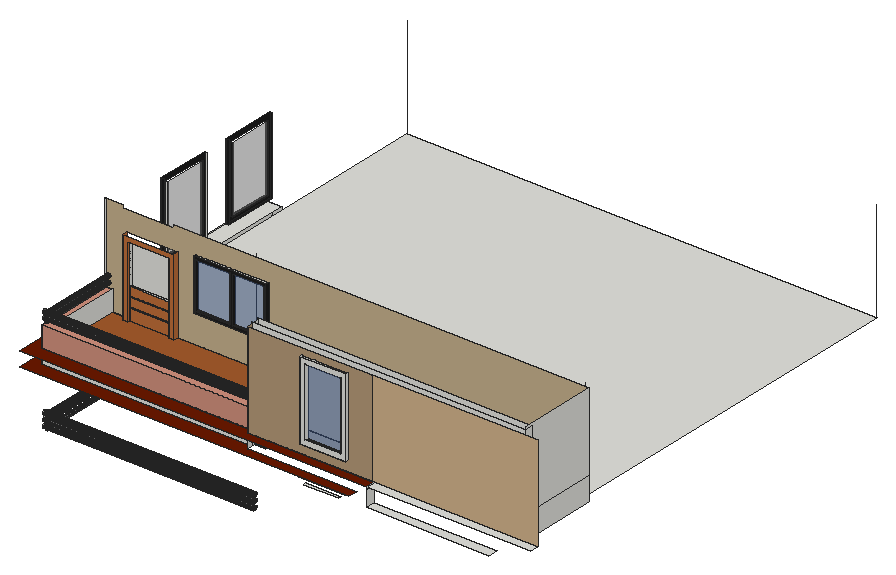
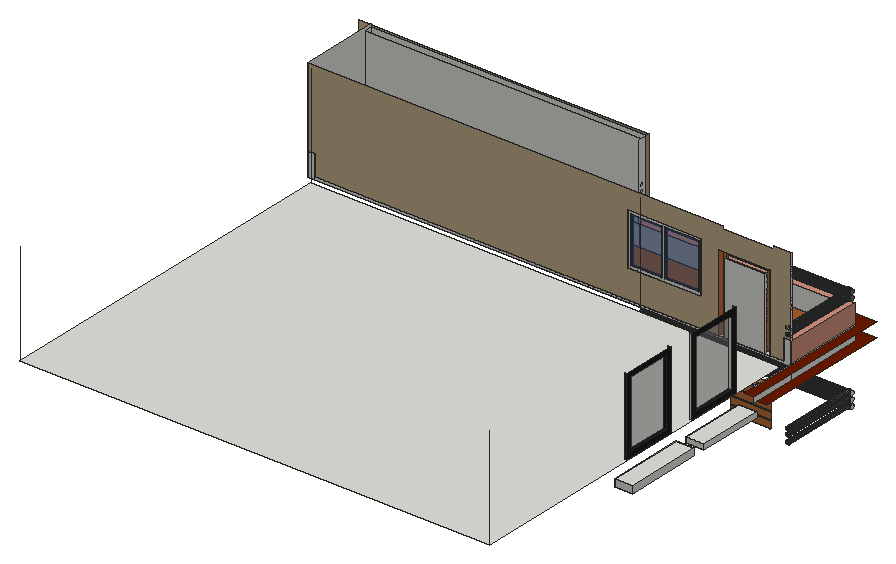
# SketchUp Ruby script. Lengths in inches.
U = 1.inch
M = Sketchup.active_model
def pt(a) = Geom::Point3d.new(a.map { |v| v * U })
def face(e, loops, mat)
  f = e.add_face(loops[0].map { |a| pt(a) })
  loops[1..].each { |l| e.add_face(l.map { |a| pt(a) }).erase! }
  f.material = f.back_material = mat if mat
  f
end
# faces: each face lists its corners as indices into pts; further lists are holes
def faces(e, pts, list, mat = nil) = list.each { |f| face(e, (f[0].is_a?(Array) ? f : [f]).map { |l| l.map { |i| pts[i] } }, mat) }
# xy, xz, yz: faces in a plane at the given z, y or x. An outline is a flat list of corners, or four numbers for a rectangle; further outlines are holes
def ring(l) = l.size == 4 ? [[l[0], l[1]], [l[2], l[1]], [l[2], l[3]], [l[0], l[3]]] : l.each_slice(2).to_a
def flat(e, list, mat, &to3) = list.each { |f| face(e, (f[0].is_a?(Array) ? f : [f]).map { |l| ring(l).map { |u, v| to3.(u, v) } }, mat) }
def xy(e, z, list, mat = nil) = flat(e, list, mat) { |x, y| [x, y, z] }
def xz(e, y, list, mat = nil) = flat(e, list, mat) { |x, z| [x, y, z] }
def yz(e, x, list, mat = nil) = flat(e, list, mat) { |y, z| [x, y, z] }
def lines(e, pts, list) = list.each { |a, b| e.add_line(pt(pts[a]), pt(pts[b])) }
# prism: a flat outline (further loops are holes) pulled along v
def prism(e, loops, v, mat = nil)
  f = face(e, loops, mat); d = Geom::Vector3d.new(v.map { |x| x * U })
  f.pushpull(f.normal.samedirection?(d) ? d.length : -d.length)
end
def box(e, o, s, mat = nil) = prism(e, [[o, [o[0] + s[0], o[1], o[2]], [o[0] + s[0], o[1] + s[1], o[2]], [o[0], o[1] + s[1], o[2]]]], [0, 0, s[2]], mat)
def at(x, y, z, deg = 0) = Geom::Transformation.translation(pt([x, y, z])) * Geom::Transformation.rotation(ORIGIN, Z_AXIS, deg.degrees)
def axes(o, x, y, z) = Geom::Transformation.new([*x, 0, *y, 0, *z, 0, *pt(o).to_a, 1])
def part(name) = M.definitions.add(name)
# library, detail: a bought-in or finely detailed component or shape, given as its bounding box
def library(name, o, s) = part(name).tap { |d| box(d.entities, o, s) }
def detail(e, o, s) = box(e.add_group.entities, o, s)
def put(e, d, t, mat = nil) = e.add_instance(d, t).tap { |i| i.material = mat if mat }
def group(e, t, mat = nil) = e.add_group.tap { |g| g.transformation = t; g.material = mat if mat }.entities
root = M.entities
M.materials.add("[0032_Moccasin]").color = [198, 177, 141]
M.materials.add("[0035_Tan]").color = [181, 154, 120]
M.materials.add("[0035_Tan]1").color = [210, 180, 140]
M.materials.add("[0134_DimGray]").color = [105, 105, 105]
M.materials.add("[Color B02]").color = [209, 145, 125]
M.materials.add("[Color B07]").color = [107, 26, 0]
M.materials.add("[Color M08]").color = [30, 30, 30]
M.materials.add("[Translucent Glass Blue]").color = [61, 91, 145]
M.materials["[Translucent Glass Blue]"].alpha = 0.5
M.materials.add("[Translucent Glass Gray]").color = [128, 128, 128]
M.materials["[Translucent Glass Gray]"].alpha = 0.5
M.materials.add("[Wood Square Tile 01]").color = [164, 91, 44]
M.materials.add("[Wood Veneer 01]").color = [191, 111, 58]
xy(root,293.5,[[141.33,116.9375,227.02,119.9375]],"[Color M08]")
xy(root,296.5,[[144.33,116.9375,184.18,119.9375],[187.18,116.9375,224.02,119.9375]],"[Color M08]")
xy(root,333,[[61.4,116.9375,109.4,119.9375]])
xy(root,333,[[61.4,113.9375,109.4,116.9375]],"[Wood Veneer 01]")
xy(root,339,[[55.4,113.9375,115.4,119.9375]],"[Wood Veneer 01]")
xy(root,342.9,[[350.26,17.9375,391.95,20.9375]])
xy(root,348.9,[[344.26,17.9375,397.95,20.9375]])
xy(root,350.47,[[430.625,9.86,574.78,20.9375]])
xy(root,351.1875,[[144.33,116.9375,184.18,119.9375],[187.18,116.9375,224.02,119.9375]],"[Color M08]")
xy(root,351.43,[[31.875,209.04,34.875,261.16],[31.875,307.48,34.875,359.6]],"[Color M08]")
xy(root,354.1875,[[141.33,116.9375,227.02,119.9375]],"[Color M08]")
xy(root,355.125,[[23.625,9.86,23.625,170.67,34.875,170.67,34.875,26.9375,282.125,26.9375,282.125,20.9375,410.07,20.9375,410.07,9.86]],"[Color B07]")
xy(root,357.43,[[13.875,198.04,13.875,275.26,34.875,275.26,34.875,267.16,31.875,267.16,31.875,203.04,34.875,203.04,34.875,198.04],[31.875,203.04,34.875,203.1],[31.875,203.1,34.875,267.16],[13.875,289.98,13.875,380.29,34.875,380.29,34.875,365.6,31.875,365.6,31.875,301.48,34.875,301.48,34.875,289.98],[31.875,301.48,34.875,365.6]])
xy(root,363.74,[[13.875,198.04,34.875,275.26]])
xy(root,365.49,[[13.875,289.98,34.875,380.29]])
xy(root,369,[[34.875,26.9375,34.875,119.9375,604.125,119.9375,604.125,35.9375,282.125,35.9375,282.125,26.9375],[282.125,26.9375,604.125,35.9375],[43.875,125.9375,595.125,552.98]])
xy(root,372,[[430.625,9.86,623,20.9375],[60.43,113.9375,66.43,119.9375],[114.43,113.9375,120.43,119.9375],[66.43,116.9375,114.43,119.9375]])
xy(root,372,[[23.625,9.86,430.625,9.86,430.625,20.9375,282.125,20.9375,282.125,26.9375,34.875,26.9375,34.875,189.6875,23.625,189.6875]],"[Color B07]")
xy(root,372,[[43.875,35.9375,595.125,35.9375,595.125,119.9375,120.43,119.9375,120.43,113.9375,114.43,113.9375,114.43,116.9375,66.43,116.9375,66.43,113.9375,60.43,113.9375,60.43,119.9375,43.875,119.9375]],"[Wood Square Tile 01]")
xy(root,380.37,[[31.875,206.29,34.875,270.41]])
xy(root,380.37,[[31.875,301.48,34.875,365.6]],"[Color M08]")
xy(root,384.33,[[346.1,17.9375,399.78,20.9375]])
xy(root,386.37,[[31.875,212.29,34.875,264.41],[31.875,307.48,34.875,359.6]],"[Color M08]")
xy(root,390.33,[[352.1,17.9375,393.78,20.9375]])
xy(root,396,[[282.125,26.9375,604.125,35.9375],[595.125,35.9375,604.125,119.9375]])
xy(root,396,[[34.875,26.9375,282.125,26.9375,282.125,35.9375,43.875,35.9375,43.875,119.9375,34.875,119.9375]],"[Color B02]")
xy(root,406.125,[[141.33,116.9375,227.02,119.9375]])
xy(root,409.125,[[144.33,116.9375,184.18,119.9375],[187.18,116.9375,224.02,119.9375]],"[Color M08]")
xz(root,17.9375,[[[346.1,384.33,399.78,476.15],[352.1,390.33,393.78,470.15]]])
xz(root,20.9375,[[282.125,369,430.625,372],[[346.1,384.33,399.78,476.15],[352.1,390.33,393.78,470.15]]])
xz(root,20.9375,[[[282.125,372,427.625,483.875],[346.1,384.33,399.78,476.15]]],"[0035_Tan]")
xz(root,20.9375,[[427.625,372,623,483.875]],"[0035_Tan]1")
xz(root,20.9375,[[352.1,390.33,393.78,470.15]],"[Translucent Glass Blue]")
xz(root,26.9375,[[34.875,355.125,282.125,369],[34.875,369,282.125,372],[282.125,369,604.125,396],[282.125,396,604.125,485.875]])
xz(root,26.9375,[[34.875,372,282.125,396]],"[Color B02]")
xz(root,29.25,[[39.51,399.11,40.12,399.19,40.69,399.43,41.1875,399.81,41.5625,400.3,41.8,400.87,41.88,401.49,41.8,402.1,41.5625,402.67,41.1875,403.17,40.69,403.54,40.12,403.78,39.51,403.86,38.89,403.78,38.32,403.54,37.83,403.17,37.45,402.67,37.21,402.1,37.13,401.49,37.21,400.87,37.45,400.3,37.83,399.81,38.32,399.43,38.89,399.19]])
xz(root,35.9375,[[43.875,372,282.125,396],[282.125,372,595.125,396],[282.125,396,604.125,485.875]])
xz(root,113.9375,[[60.43,372,66.43,372,66.43,456,114.43,456,114.43,372,120.43,372,120.43,462,60.43,462]],"[Wood Veneer 01]")
xz(root,116.9375,[[61.4,292.58,109.4,293.56],[61.4,301.83,109.4,302.81],[61.4,311.08,109.4,312.06],[61.4,320.33,109.4,321.31],[66.43,385.34,114.43,387.06],
  [66.43,396.78,114.43,398.5],[66.43,408.22,114.43,409.93]])
xz(root,116.9375,[[[141.33,293.5,227.02,354.1875],[144.33,296.5,184.18,351.1875],[187.18,296.5,224.02,351.1875]],[[141.33,406.125,227.02,466.8125],[144.33,409.125,184.18,463.8125],[187.18,409.125,224.02,463.8125]]],"[Color M08]")
xz(root,116.9375,[[61.4,293.56,109.4,301.83],[61.4,302.81,109.4,311.08],[61.4,312.06,109.4,320.33],[61.4,321.31,109.4,333],[66.43,372,114.43,385.34],
  [66.43,387.06,114.43,396.78],[66.43,398.5,114.43,408.22]],"[Wood Veneer 01]")
xz(root,119.9375,[[[141.33,293.5,227.02,354.1875],[144.33,296.5,184.18,351.1875],[187.18,296.5,224.02,351.1875]],[34.875,369,35.6,396],[35.6,369,60.43,369,60.43,372,43.875,372,43.875,396,35.6,396],[60.43,369,120.43,372],[120.43,369,595.125,372],
  [595.125,369,604.125,396],[66.43,372,114.43,456],[34.875,396,35.6,489],[[141.33,406.125,227.02,466.8125],[144.33,409.125,184.18,463.8125],[187.18,409.125,224.02,463.8125]]])
xz(root,119.9375,[[[43.875,372,60.43,372,60.43,462,120.43,462,120.43,372,595.125,372,595.125,396,604.125,396,604.125,489,116.21,489,116.21,486,56.21,486,56.21,489,35.6,489,35.6,396,43.875,396],[141.33,406.125,227.02,466.8125],[39.51,399.11,38.89,399.19,38.32,399.43,37.83,399.81,37.45,400.3,37.21,400.87,37.13,401.49,37.21,402.1,37.45,402.67,37.83,403.17,38.32,403.54,38.89,403.78,39.51,403.86,40.12,403.78,40.69,403.54,41.1875,403.17,41.5625,402.67,41.8,402.1,41.88,401.49,41.8,400.87,41.5625,400.3,41.1875,399.81,40.69,399.43,40.12,399.19]]],"[0032_Moccasin]")
xz(root,119.9375,[[144.33,296.5,184.18,351.1875],[187.18,296.5,224.02,351.1875],[144.33,409.125,184.18,463.8125],[187.18,409.125,224.02,463.8125]],"[Translucent Glass Blue]")
xz(root,198.04,[[13.875,357.43,34.875,363.74]])
xz(root,206.29,[[31.875,380.37,34.875,470.8]],"[Color M08]")
xz(root,212.29,[[31.875,386.37,34.875,464.8]])
xz(root,264.41,[[31.875,386.37,34.875,464.8]],"[Color M08]")
xz(root,270.41,[[31.875,380.37,34.875,470.8]])
xz(root,275.26,[[13.875,357.43,34.875,363.74]])
xz(root,289.98,[[13.875,357.43,34.875,365.49]])
xz(root,301.48,[[31.875,380.37,34.875,470.8]],"[Color M08]")
xz(root,307.48,[[31.875,386.37,34.875,464.8]],"[Color M08]")
xz(root,359.6,[[31.875,386.37,34.875,464.8]],"[Color M08]")
xz(root,365.6,[[31.875,380.37,34.875,470.8]],"[Color M08]")
xz(root,380.29,[[13.875,357.43,34.875,365.49]])
yz(root,13.875,[[198.04,357.43,275.26,363.74],[289.98,357.43,380.29,365.49]])
yz(root,31.875,[[[206.29,380.37,270.41,470.8],[212.29,386.37,264.41,464.8]],[[301.48,380.37,365.6,470.8],[307.48,386.37,359.6,464.8]]],"[Color M08]")
yz(root,34.875,[[31.46,285.87,30.85,285.95,30.27,286.1875,29.78,286.5625,29.4,287.06,29.17,287.63,29.09,288.24,29.17,288.86,29.4,289.43,29.78,289.92,30.27,290.3,30.85,290.54,31.46,290.62,32.08,290.54,32.65,290.3,33.14,289.92,33.52,289.43,33.76,288.86,33.84,288.24,33.76,287.63,33.52,287.06,33.14,286.5625,32.65,286.1875,32.08,285.95],[31.46,292.87,30.85,292.95,30.27,293.1875,29.78,293.5625,29.4,294.06,29.17,294.63,29.09,295.24,29.17,295.86,29.4,296.43,29.78,296.92,30.27,297.3,30.85,297.54,31.46,297.62,32.08,297.54,32.65,297.3,33.14,296.92,33.52,296.43,33.76,295.86,33.84,295.24,33.76,294.63,33.52,294.06,33.14,293.5625,32.65,293.1875,32.08,292.95],[31.46,299.87,30.85,299.95,30.27,300.1875,29.78,300.5625,29.4,301.06,29.17,301.63,29.09,302.24,29.17,302.86,29.4,303.43,29.78,303.92,30.27,304.3,30.85,304.54,31.46,304.62,32.08,304.54,32.65,304.3,33.14,303.92,33.52,303.43,33.76,302.86,33.84,302.24,33.76,301.63,33.52,301.06,33.14,300.5625,32.65,300.1875,32.08,299.95],[26.9375,355.125,119.9375,369],[119.9375,355.125,175.54,369],
  [198.04,357.43,203.1,363.74],[203.1,357.43,275.26,363.74],[289.98,357.43,365.6,365.49],[365.6,357.43,380.29,365.49],[26.9375,369,119.9375,372],
  [119.9375,369,175.54,372]])
yz(root,34.875,[[31.46,399.68,30.85,399.76,30.27,400,29.78,400.375,29.4,400.87,29.17,401.44,29.09,402.06,29.17,402.67,29.4,403.24,29.78,403.73,30.27,404.11,30.85,404.35,31.46,404.43,32.08,404.35,32.65,404.11,33.14,403.73,33.52,403.24,33.76,402.67,33.84,402.06,33.76,401.44,33.52,400.87,33.14,400.375,32.65,400,32.08,399.76],[31.46,406.37,30.85,406.45,30.27,406.6875,29.78,407.0625,29.4,407.56,29.17,408.13,29.09,408.74,29.17,409.36,29.4,409.93,29.78,410.42,30.27,410.8,30.85,411.04,31.46,411.12,32.08,411.04,32.65,410.8,33.14,410.42,33.52,409.93,33.76,409.36,33.84,408.74,33.76,408.13,33.52,407.56,33.14,407.0625,32.65,406.6875,32.08,406.45]],"[0134_DimGray]")
yz(root,34.875,[[26.9375,372,119.9375,396]],"[Color B02]")
yz(root,34.875,[[212.29,386.37,264.41,464.8],[307.48,386.37,359.6,464.8]],"[Translucent Glass Gray]")
yz(root,43.875,[[35.9375,372,119.9375,396]])
yz(root,60.43,[[113.9375,372,119.9375,462]],"[Wood Veneer 01]")
yz(root,66.43,[[116.9375,372,119.9375,456]])
yz(root,66.43,[[113.9375,372,116.9375,456]],"[Wood Veneer 01]")
yz(root,114.43,[[116.9375,372,119.9375,456]])
yz(root,114.43,[[113.9375,372,116.9375,456]],"[Wood Veneer 01]")
yz(root,120.43,[[113.9375,372,119.9375,462]],"[Wood Veneer 01]")
yz(root,141.33,[[116.9375,293.5,119.9375,354.1875]])
yz(root,141.33,[[116.9375,406.125,119.9375,466.8125]],"[Color M08]")
yz(root,144.33,[[116.9375,296.5,119.9375,351.1875],[116.9375,409.125,119.9375,463.8125]],"[Color M08]")
yz(root,184.18,[[116.9375,296.5,119.9375,351.1875],[116.9375,409.125,119.9375,463.8125]],"[Color M08]")
yz(root,187.18,[[116.9375,296.5,119.9375,351.1875],[116.9375,409.125,119.9375,463.8125]],"[Color M08]")
yz(root,224.02,[[116.9375,296.5,119.9375,351.1875],[116.9375,409.125,119.9375,463.8125]],"[Color M08]")
yz(root,227.02,[[116.9375,293.5,119.9375,354.1875],[116.9375,406.125,119.9375,466.8125]],"[Color M08]")
yz(root,282.125,[[20.9375,355.125,26.9375,369],[26.9375,355.125,35.9375,369],[20.9375,369,26.9375,372],[[26.9375,396,35.9375,483.875],[31.46,399.68,32.08,399.76,32.65,400,33.14,400.375,33.52,400.87,33.76,401.44,33.84,402.06,33.76,402.67,33.52,403.24,33.14,403.73,32.65,404.11,32.08,404.35,31.46,404.43,30.85,404.35,30.27,404.11,29.78,403.73,29.4,403.24,29.17,402.67,29.09,402.06,29.17,401.44,29.4,400.87,29.78,400.375,30.27,400,30.85,399.76],[31.46,406.37,32.08,406.45,32.65,406.6875,33.14,407.0625,33.52,407.56,33.76,408.13,33.84,408.74,33.76,409.36,33.52,409.93,33.14,410.42,32.65,410.8,32.08,411.04,31.46,411.12,30.85,411.04,30.27,410.8,29.78,410.42,29.4,409.93,29.17,409.36,29.09,408.74,29.17,408.13,29.4,407.56,29.78,407.0625,30.27,406.6875,30.85,406.45],[31.46,413.06,32.08,413.14,32.65,413.375,33.14,413.75,33.52,414.24,33.76,414.82,33.84,415.43,33.76,416.04,33.52,416.62,33.14,417.11,32.65,417.49,32.08,417.72,31.46,417.81,30.85,417.72,30.27,417.49,29.78,417.11,29.4,416.62,29.17,416.04,29.09,415.43,29.17,414.82,29.4,414.24,29.78,413.75,30.27,413.375,30.85,413.14],[31.46,419.74,32.08,419.82,32.65,420.0625,33.14,420.4375,33.52,420.93,33.76,421.5,33.84,422.12,33.76,422.73,33.52,423.31,33.14,423.8,32.65,424.17,32.08,424.41,31.46,424.49,30.85,424.41,30.27,424.17,29.78,423.8,29.4,423.31,29.17,422.73,29.09,422.12,29.17,421.5,29.4,420.93,29.78,420.4375,30.27,420.0625,30.85,419.82],[31.46,426.43,32.08,426.51,32.65,426.75,33.14,427.125,33.52,427.62,33.76,428.19,33.84,428.81,33.76,429.42,33.52,429.99,33.14,430.48,32.65,430.86,32.08,431.1,31.46,431.18,30.85,431.1,30.27,430.86,29.78,430.48,29.4,429.99,29.17,429.42,29.09,428.81,29.17,428.19,29.4,427.62,29.78,427.125,30.27,426.75,30.85,426.51],[31.46,433.12,32.08,433.2,32.65,433.4375,33.14,433.8125,33.52,434.31,33.76,434.88,33.84,435.49,33.76,436.11,33.52,436.68,33.14,437.17,32.65,437.55,32.08,437.79,31.46,437.87,30.85,437.79,30.27,437.55,29.78,437.17,29.4,436.68,29.17,436.11,29.09,435.49,29.17,434.88,29.4,434.31,29.78,433.8125,30.27,433.4375,30.85,433.2]]])
yz(root,282.125,[[20.9375,372,26.9375,483.875]],"[0035_Tan]")
yz(root,346.1,[[17.9375,384.33,20.9375,476.15]])
yz(root,352.1,[[17.9375,390.33,20.9375,470.15]])
yz(root,393.78,[[17.9375,390.33,20.9375,470.15]])
yz(root,399.78,[[17.9375,384.33,20.9375,476.15]])
yz(root,430.625,[[9.86,350.47,20.9375,369],[9.86,369,20.9375,372]])
yz(root,595.125,[[35.9375,372,119.9375,396]])
yz(root,604.125,[[26.9375,369,119.9375,396],[26.9375,396,35.9375,485.875],[35.9375,396,35.9375,485.875,26.9375,485.875,26.9375,489,119.9375,489,119.9375,396]])
p = [[38.98,119.9375,285.88],[39.53,119.9375,285.8125],[39.53,29.17,285.8125],[38.98,29.17,285.88],[40.08,119.9375,285.88],[40.08,29.17,285.88],
  [38.47,119.9375,286.1],[38.47,29.17,286.1],[40.59,119.9375,286.1],[40.59,29.17,286.1],[282.125,30.85,285.95],[282.125,30.27,286.1875],
  [34.875,30.27,286.1875],[34.875,30.85,285.95],[282.125,31.46,285.87],[34.875,31.46,285.87],[282.125,32.08,285.95],[34.875,32.08,285.95],
  [282.125,32.65,286.1875],[34.875,32.65,286.1875],[38.03,119.9375,286.43],[38.03,29.17,286.43],[41.03,119.9375,286.43],[41.03,29.17,286.43],
  [282.125,29.78,286.5625],[34.875,29.78,286.5625],[282.125,33.14,286.5625],[34.875,33.14,286.5625],[37.69,119.9375,286.875],[37.69,29.17,286.875],
  [41.37,119.9375,286.875],[41.37,29.17,286.875],[282.125,29.4,287.06],[34.875,29.4,287.06],[282.125,33.52,287.06],[34.875,33.52,287.06],
  [37.48,119.9375,287.39],[37.48,29.17,287.39],[41.58,119.9375,287.39],[41.58,29.17,287.39],[282.125,29.17,287.63],[41.62,29.17,287.63],
  [37.45,29.17,287.63],[34.875,29.17,287.63],[282.125,33.76,287.63],[34.875,33.76,287.63],[37.41,119.9375,287.9375],[37.41,29.17,287.9375],
  [41.66,119.9375,287.9375],[41.66,29.17,287.9375],[282.125,29.09,288.24],[34.875,29.09,288.24],[282.125,33.84,288.24],[34.875,33.84,288.24],
  [37.48,119.9375,288.49],[37.41,29.17,287.94],[37.43,29.17,288.13],[37.48,29.17,288.49],[41.58,119.9375,288.49],[41.58,29.17,288.49],
  [41.63,29.17,288.13],[41.66,29.17,287.94],[282.125,29.17,288.86],[41.43,29.17,288.86],[37.63,29.17,288.86],[34.875,29.17,288.86],
  [282.125,33.76,288.86],[34.875,33.76,288.86],[37.69,119.9375,289],[37.69,29.17,289],[41.37,119.9375,289],[41.37,29.17,289],
  [282.125,29.4,289.43],[34.875,29.4,289.43],[282.125,33.52,289.43],[34.875,33.52,289.43],[38.03,119.9375,289.4375],[37.82,29.17,289.17],
  [37.97,29.17,289.36],[38.03,29.17,289.4375],[41.03,119.9375,289.4375],[41.03,29.17,289.4375],[41.1,29.17,289.36],[41.24,29.17,289.17],
  [38.47,119.9375,289.78],[38.47,29.17,289.78],[40.59,119.9375,289.78],[40.59,29.17,289.78],[282.125,29.78,289.92],[34.875,29.78,289.92],
  [282.125,33.14,289.92],[34.875,33.14,289.92],[38.98,119.9375,289.99],[38.98,29.17,289.99],[40.08,119.9375,289.99],[40.08,29.17,289.99],
  [282.125,30.27,290.3],[34.875,30.27,290.3],[282.125,32.65,290.3],[34.875,32.65,290.3],[39.53,119.9375,290.0625],[39.53,29.17,290.0625],
  [282.125,30.85,290.54],[34.875,30.85,290.54],[282.125,32.08,290.54],[34.875,32.08,290.54],[282.125,31.46,290.62],[34.875,31.46,290.62],
  [282.125,30.85,292.95],[282.125,30.27,293.1875],[34.875,30.27,293.1875],[34.875,30.85,292.95],[282.125,31.46,292.87],[34.875,31.46,292.87],
  [282.125,32.08,292.95],[34.875,32.08,292.95],[282.125,32.65,293.1875],[34.875,32.65,293.1875],[282.125,29.78,293.5625],[34.875,29.78,293.5625],
  [282.125,33.14,293.5625],[34.875,33.14,293.5625],[282.125,29.4,294.06],[34.875,29.4,294.06],[282.125,33.52,294.06],[34.875,33.52,294.06],
  [38.98,119.9375,294.01],[39.53,119.9375,293.9375],[39.53,29.17,293.9375],[38.98,29.17,294.01],[40.08,119.9375,294.01],[40.08,29.17,294.01],
  [38.47,119.9375,294.22],[38.47,29.17,294.22],[40.59,119.9375,294.22],[40.59,29.17,294.22],[282.125,29.17,294.63],[41.09,29.17,294.63],
  [37.98,29.17,294.63],[34.875,29.17,294.63],[282.125,33.76,294.63],[34.875,33.76,294.63],[38.03,119.9375,294.56],[38.03,29.17,294.56],
  [41.03,119.9375,294.56],[41.03,29.17,294.56],[282.125,29.09,295.24],[34.875,29.09,295.24],[37.69,119.9375,295],[37.69,29.17,295],
  [41.37,119.9375,295],[41.37,29.17,295],[282.125,33.84,295.24],[34.875,33.84,295.24],[37.48,119.9375,295.51],[37.48,29.17,295.51],
  [41.58,119.9375,295.51],[41.58,29.17,295.51],[282.125,29.17,295.86],[41.63,29.17,295.86],[37.43,29.17,295.86],[34.875,29.17,295.86],
  [282.125,33.76,295.86],[34.875,33.76,295.86],[37.41,119.9375,296.0625],[37.45,29.17,295.75],[37.41,29.17,296.0625],[41.66,119.9375,296.0625],
  [41.66,29.17,296.0625],[41.62,29.17,295.75],[282.125,29.4,296.43],[34.875,29.4,296.43],[282.125,33.52,296.43],[34.875,33.52,296.43],
  [37.48,119.9375,296.61],[37.41,29.17,296.07],[37.43,29.17,296.25],[37.48,29.17,296.61],[41.58,119.9375,296.61],[41.58,29.17,296.61],
  [41.63,29.17,296.25],[41.66,29.17,296.07],[282.125,29.78,296.92],[34.875,29.78,296.92],[282.125,33.14,296.92],[34.875,33.14,296.92],
  [37.69,119.9375,297.125],[37.63,29.17,296.98],[37.69,29.17,297.125],[41.37,119.9375,297.125],[41.37,29.17,297.125],[41.43,29.17,296.98],
  [282.125,30.27,297.3],[34.875,30.27,297.3],[282.125,32.65,297.3],[34.875,32.65,297.3],[38.03,119.9375,297.5625],[37.82,29.17,297.29],
  [37.97,29.17,297.48],[38.03,29.17,297.5625],[41.03,119.9375,297.5625],[41.03,29.17,297.5625],[41.1,29.17,297.48],[41.24,29.17,297.29],
  [282.125,30.85,297.54],[34.875,30.85,297.54],[282.125,32.08,297.54],[34.875,32.08,297.54],[282.125,31.46,297.62],[34.875,31.46,297.62],
  [38.47,119.9375,297.9],[38.47,29.17,297.9],[40.59,119.9375,297.9],[40.59,29.17,297.9],[38.98,119.9375,298.11],[38.98,29.17,298.11],
  [40.08,119.9375,298.11],[40.08,29.17,298.11],[39.53,119.9375,298.1875],[39.53,29.17,298.1875],[282.125,30.85,299.95],[282.125,30.27,300.1875],
  [34.875,30.27,300.1875],[34.875,30.85,299.95],[282.125,31.46,299.87],[34.875,31.46,299.87],[282.125,32.08,299.95],[34.875,32.08,299.95],
  [282.125,32.65,300.1875],[34.875,32.65,300.1875],[38.98,119.9375,300.32],[39.53,119.9375,300.25],[39.53,29.17,300.25],[38.98,29.17,300.32],
  [40.08,119.9375,300.32],[40.08,29.17,300.32],[282.125,29.78,300.5625],[34.875,29.78,300.5625],[282.125,33.14,300.5625],[34.875,33.14,300.5625],
  [38.47,119.9375,300.53],[38.47,29.17,300.53],[40.59,119.9375,300.53],[40.59,29.17,300.53],[38.03,119.9375,300.87],[38.03,29.17,300.87],
  [41.03,119.9375,300.87],[41.03,29.17,300.87],[282.125,29.4,301.06],[34.875,29.4,301.06],[282.125,33.52,301.06],[34.875,33.52,301.06],
  [37.69,119.9375,301.3125],[37.98,29.17,300.94],[37.69,29.17,301.3125],[41.37,119.9375,301.3125],[41.37,29.17,301.3125],[41.09,29.17,300.94],
  [282.125,29.17,301.63],[41.5,29.17,301.63],[37.56,29.17,301.63],[34.875,29.17,301.63],[282.125,33.76,301.63],[34.875,33.76,301.63],
  [37.48,119.9375,301.82],[37.48,29.17,301.82],[41.58,119.9375,301.82],[41.58,29.17,301.82],[282.125,29.09,302.24],[34.875,29.09,302.24],
  [282.125,33.84,302.24],[34.875,33.84,302.24],[37.41,119.9375,302.375],[37.45,29.17,302.07],[37.43,29.17,302.17],[37.41,29.17,302.375],
  [41.66,119.9375,302.375],[41.66,29.17,302.375],[41.63,29.17,302.17],[41.62,29.17,302.07],[282.125,29.17,302.86],[41.59,29.17,302.86],
  [37.47,29.17,302.86],[34.875,29.17,302.86],[282.125,33.76,302.86],[34.875,33.76,302.86],[37.48,119.9375,302.92],[37.41,29.17,302.38],
  [37.43,29.17,302.57],[37.48,29.17,302.92],[41.58,119.9375,302.92],[41.58,29.17,302.92],[41.63,29.17,302.57],[41.66,29.17,302.38],
  [282.125,29.4,303.43],[34.875,29.4,303.43],[37.69,119.9375,303.4375],[37.63,29.17,303.29],[37.69,29.17,303.4375],[41.37,119.9375,303.4375],
  [41.37,29.17,303.4375],[41.43,29.17,303.29],[282.125,33.52,303.43],[34.875,33.52,303.43],[38.03,119.9375,303.875],[37.82,29.17,303.61],
  [37.97,29.17,303.79],[38.03,29.17,303.875],[41.03,119.9375,303.875],[41.03,29.17,303.875],[41.1,29.17,303.79],[41.24,29.17,303.61],
  [282.125,29.78,303.92],[34.875,29.78,303.92],[282.125,33.14,303.92],[34.875,33.14,303.92],[38.47,119.9375,304.21],[38.47,29.17,304.21],
  [40.59,119.9375,304.21],[40.59,29.17,304.21],[282.125,30.27,304.3],[34.875,30.27,304.3],[282.125,32.65,304.3],[34.875,32.65,304.3],
  [38.98,119.9375,304.43],[38.98,29.17,304.43],[40.08,119.9375,304.43],[40.08,29.17,304.43],[282.125,30.85,304.54],[34.875,30.85,304.54],
  [282.125,32.08,304.54],[34.875,32.08,304.54],[39.53,119.9375,304.5],[39.53,29.17,304.5],[282.125,31.46,304.62],[34.875,31.46,304.62],
  [38.89,119.9375,399.19],[39.51,119.9375,399.11],[39.51,29.25,399.11],[38.89,29.25,399.19],[40.12,119.9375,399.19],[40.12,29.25,399.19],
  [38.32,119.9375,399.43],[38.32,29.25,399.43],[40.69,119.9375,399.43],[40.69,29.25,399.43],[37.83,119.9375,399.81],[37.83,29.25,399.81],
  [41.1875,119.9375,399.81],[41.1875,29.25,399.81],[282.125,31.46,399.68],[282.125,30.85,399.76],[34.875,30.85,399.76],[34.875,31.46,399.68],
  [282.125,32.08,399.76],[34.875,32.08,399.76],[37.45,119.9375,400.3],[37.45,29.25,400.3],[41.5625,119.9375,400.3],[41.5625,29.25,400.3],
  [282.125,30.27,400],[34.875,30.27,400],[282.125,32.65,400],[34.875,32.65,400],[282.125,29.78,400.375],[34.875,29.78,400.375],
  [282.125,33.14,400.375],[34.875,33.14,400.375],[37.21,119.9375,400.87],[37.21,29.25,400.87],[41.8,119.9375,400.87],[41.8,29.25,400.87],
  [282.125,29.4,400.87],[34.875,29.4,400.87],[282.125,33.52,400.87],[34.875,33.52,400.87],[282.125,29.17,401.44],[34.875,29.17,401.44],
  [37.13,119.9375,401.49],[37.13,29.25,401.49],[41.88,119.9375,401.49],[41.88,29.25,401.49],[282.125,33.76,401.44],[34.875,33.76,401.44],
  [282.125,29.09,402.06],[34.875,29.09,402.06],[282.125,33.84,402.06],[34.875,33.84,402.06],[37.21,119.9375,402.1],[37.21,29.25,402.1],
  [41.8,119.9375,402.1],[41.8,29.25,402.1],[282.125,29.17,402.67],[34.875,29.17,402.67],[37.45,119.9375,402.67],[37.45,29.25,402.67],
  [41.5625,119.9375,402.67],[41.5625,29.25,402.67],[282.125,33.76,402.67],[34.875,33.76,402.67],[282.125,29.4,403.24],[34.875,29.4,403.24],
  [37.83,119.9375,403.17],[37.83,29.25,403.17],[41.1875,119.9375,403.17],[41.1875,29.25,403.17],[282.125,33.52,403.24],[34.875,33.52,403.24],
  [38.32,119.9375,403.54],[38.32,29.25,403.54],[40.69,119.9375,403.54],[40.69,29.25,403.54],[282.125,29.78,403.73],[34.875,29.78,403.73],
  [282.125,33.14,403.73],[34.875,33.14,403.73],[38.89,119.9375,403.78],[38.89,29.25,403.78],[40.12,119.9375,403.78],[40.12,29.25,403.78],
  [282.125,30.27,404.11],[34.875,30.27,404.11],[282.125,32.65,404.11],[34.875,32.65,404.11],[39.51,119.9375,403.86],[39.51,29.25,403.86],
  [282.125,30.85,404.35],[34.875,30.85,404.35],[282.125,32.08,404.35],[34.875,32.08,404.35],[282.125,31.46,404.43],[34.875,31.46,404.43],
  [282.125,30.85,406.45],[282.125,30.27,406.6875],[34.875,30.27,406.6875],[34.875,30.85,406.45],[282.125,31.46,406.37],[34.875,31.46,406.37],
  [282.125,32.08,406.45],[34.875,32.08,406.45],[282.125,32.65,406.6875],[34.875,32.65,406.6875],[38.89,119.9375,406.57],[39.51,119.9375,406.49],
  [39.51,29.25,406.49],[38.89,29.25,406.57],[40.12,119.9375,406.57],[40.12,29.25,406.57],[38.32,119.9375,406.81],[38.32,29.25,406.81],
  [40.69,119.9375,406.81],[40.69,29.25,406.81],[282.125,29.78,407.0625],[34.875,29.78,407.0625],[282.125,33.14,407.0625],[34.875,33.14,407.0625],
  [37.83,119.9375,407.18],[37.83,29.25,407.18],[41.1875,119.9375,407.18],[41.1875,29.25,407.18],[282.125,29.4,407.56],[34.875,29.4,407.56],
  [282.125,33.52,407.56],[34.875,33.52,407.56],[37.45,119.9375,407.67],[37.45,29.25,407.67],[41.5625,119.9375,407.67],[41.5625,29.25,407.67],
  [282.125,29.17,408.13],[34.875,29.17,408.13],[282.125,33.76,408.13],[34.875,33.76,408.13],[37.21,119.9375,408.25],[37.21,29.25,408.25],
  [41.8,119.9375,408.25],[41.8,29.25,408.25],[282.125,29.09,408.74],[34.875,29.09,408.74],[282.125,33.84,408.74],[34.875,33.84,408.74],
  [37.13,119.9375,408.86],[37.13,29.25,408.86],[41.88,119.9375,408.86],[41.88,29.25,408.86],[282.125,29.17,409.36],[34.875,29.17,409.36],
  [282.125,33.76,409.36],[34.875,33.76,409.36],[37.21,119.9375,409.48],[37.21,29.25,409.48],[41.8,119.9375,409.48],[41.8,29.25,409.48],
  [282.125,29.4,409.93],[34.875,29.4,409.93],[282.125,33.52,409.93],[34.875,33.52,409.93],[37.45,119.9375,410.05],[37.45,29.25,410.05],
  [41.5625,119.9375,410.05],[41.5625,29.25,410.05],[37.83,119.9375,410.54],[37.83,29.25,410.54],[41.1875,119.9375,410.54],[41.1875,29.25,410.54],
  [38.32,119.9375,410.92],[38.32,29.25,410.92],[40.69,119.9375,410.92],[40.69,29.25,410.92],[38.89,119.9375,411.16],[38.89,29.25,411.16],
  [40.12,119.9375,411.16],[40.12,29.25,411.16],[39.51,119.9375,411.24],[39.51,29.25,411.24],[595.125,552.98,369],[595.125,552.98,489],
  [595.125,125.9375,369],[595.125,125.9375,489],[207.54,125.9375,369],[207.54,125.9375,489],[43.875,552.98,369],[43.875,552.98,489],
  [604.125,26.9375,372],[604.125,23.9375,372],[607.125,26.9375,372],[604.125,26.9375,369],[607.125,26.9375,369]]
faces(root,p,[[0,1,2,3],[1,4,5,2],[6,0,3,7],[4,8,9,5],[10,11,12,13],[14,10,13,15],[16,14,15,17],[18,16,17,19],
  [20,6,7,21],[8,22,23,9],[11,24,25,12],[26,18,19,27],[28,20,21,29],[22,30,31,23],[24,32,33,25],[34,26,27,35],
  [36,28,29,37],[30,38,39,31],[32,40,41,42,43,33],[44,34,35,45],[46,36,37,42,47],[38,48,49,41,39],[40,50,51,43,42,41],[52,44,45,53],
  [54,46,47,55,56,57],[48,58,59,60,61,49],[50,62,63,64,65,51],[66,52,53,67],[68,54,57,64,69],[58,70,71,63,59],[62,72,73,65,64,63],[74,66,67,75],
  [76,68,69,77,78,79],[70,80,81,82,83,71],[84,76,79,85],[80,86,87,81],[72,88,89,73],[90,74,75,91],[92,84,85,93],[86,94,95,87],
  [88,96,97,89],[98,90,91,99],[100,92,93,101],[94,100,101,95],[96,102,103,97],[104,98,99,105],[102,106,107,103],[106,104,105,107],
  [108,109,110,111],[112,108,111,113],[114,112,113,115],[116,114,115,117],[109,118,119,110],[120,116,117,121],[118,122,123,119],[124,120,121,125],
  [126,127,128,129],[127,130,131,128],[132,126,129,133],[130,134,135,131],[122,136,137,138,139,123],[140,124,125,141],[142,132,133,143],[134,144,145,135],
  [136,146,147,139,138,137],[148,142,143,138,149],[144,150,151,137,145],[152,140,141,153],[154,148,149,155],[150,156,157,151],[146,158,159,160,161,147],[162,152,153,163],
  [164,154,155,165,160,166],[156,167,168,159,169,157],[158,170,171,161,160,159],[172,162,163,173],[174,164,166,175,176,177],[167,178,179,180,181,168],[170,182,183,171],[184,172,173,185],
  [186,174,177,187,188],[178,189,190,191,179],[182,192,193,183],[194,184,185,195],[196,186,188,197,198,199],[189,200,201,202,203,190],[192,204,205,193],[206,194,195,207],
  [204,208,209,205],[208,206,207,209],[210,196,199,211],[200,212,213,201],[214,210,211,215],[212,216,217,213],[218,214,215,219],[216,218,219,217],
  [220,221,222,223],[224,220,223,225],[226,224,225,227],[228,226,227,229],[230,231,232,233],[231,234,235,232],[221,236,237,222],[238,228,229,239],
  [240,230,233,241],[234,242,243,235],[244,240,241,245],[242,246,247,243],[236,248,249,237],[250,238,239,251],[252,244,245,253,254],[246,255,256,257,247],
  [248,258,259,260,261,249],[262,250,251,263],[264,252,254,260,265],[255,266,267,259,256],[258,268,269,261,260,259],[270,262,263,271],[272,264,265,273,274,275],[266,276,277,278,279,267],
  [268,280,281,282,283,269],[284,270,271,285],[286,272,275,287,288,282,289],[276,290,291,281,292,293,277],[280,294,295,283,282,281],[296,286,289,297,298],[290,299,300,301,291],[302,284,285,303],
  [304,296,298,305,306,307],[299,308,309,310,311,300],[294,312,313,295],[314,302,303,315],[316,304,307,317],[308,318,319,309],[312,320,321,313],[322,314,315,323],
  [324,316,317,325],[318,326,327,319],[320,328,329,321],[330,322,323,331],[332,324,325,333],[326,332,333,327],[328,334,335,329],[334,330,331,335],
  [336,337,338,339],[337,340,341,338],[342,336,339,343],[340,344,345,341],[346,342,343,347],[344,348,349,345],[350,351,352,353],[354,350,353,355],
  [356,346,347,357],[348,358,359,349],[351,360,361,352],[362,354,355,363],[360,364,365,361],[366,362,363,367],[368,356,357,369],[358,370,371,359],
  [364,372,373,365],[374,366,367,375],[372,376,377,373],[378,368,369,379],[370,380,381,371],[382,374,375,383],[376,384,385,377],[386,382,383,387],
  [388,378,379,389],[380,390,391,381],[384,392,393,385],[394,388,389,395],[390,396,397,391],[398,386,387,399],[392,400,401,393],[402,394,395,403],
  [396,404,405,397],[406,398,399,407],[408,402,403,409],[404,410,411,405],[400,412,413,401],[414,406,407,415],[416,408,409,417],[410,418,419,411],
  [412,420,421,413],[422,414,415,423],[424,416,417,425],[418,424,425,419],[420,426,427,421],[428,422,423,429],[426,430,431,427],[430,428,429,431],
  [432,433,434,435],[436,432,435,437],[438,436,437,439],[440,438,439,441],[442,443,444,445],[443,446,447,444],[448,442,445,449],[446,450,451,447],
  [433,452,453,434],[454,440,441,455],[456,448,449,457],[450,458,459,451],[452,460,461,453],[462,454,455,463],[464,456,457,465],[458,466,467,459],
  [460,468,469,461],[470,462,463,471],[472,464,465,473],[466,474,475,467],[468,476,477,469],[478,470,471,479],[480,472,473,481],[474,482,483,475],
  [476,484,485,477],[486,478,479,487],[488,480,481,489],[482,490,491,483],[484,492,493,485],[494,486,487,495],[496,488,489,497],[490,498,499,491],
  [500,496,497,501],[498,502,503,499],[504,500,501,505],[502,506,507,503],[508,504,505,509],[506,510,511,507],[512,508,509,513],[510,512,513,511]],"[0134_DimGray]")
lines(root,p,[[514,515],[516,517],[518,519],[520,521],[522,523],[522,524],[525,526]])
